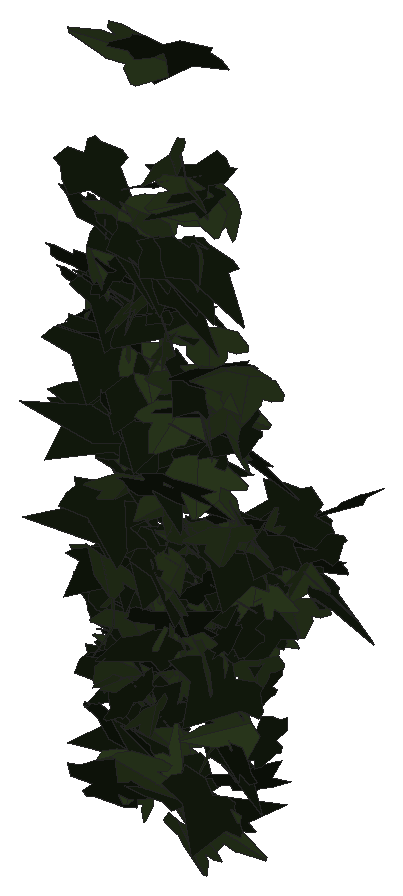
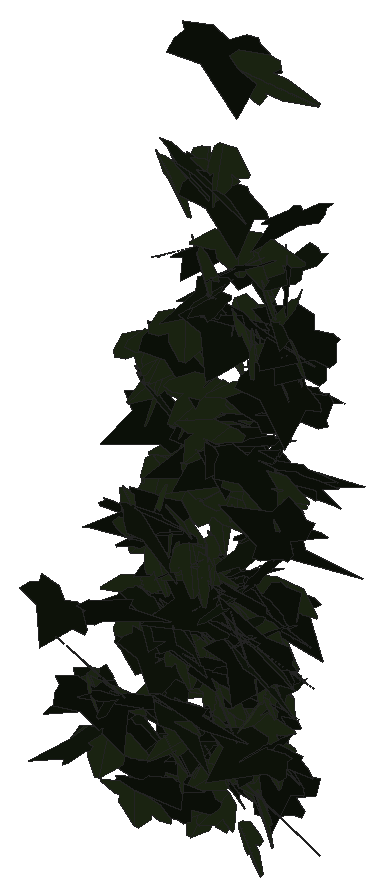
# SketchUp Ruby script. Lengths in millimetres.
U = 1.mm
M = Sketchup.active_model
def pt(a) = Geom::Point3d.new(a.map { |v| v * U })
def face(e, loops, mat)
  f = e.add_face(loops[0].map { |a| pt(a) })
  loops[1..].each { |l| e.add_face(l.map { |a| pt(a) }).erase! }
  f.material = f.back_material = mat if mat
  f
end
# faces: each face lists its corners as indices into pts; further lists are holes
def faces(e, pts, list, mat = nil) = list.each { |f| face(e, (f[0].is_a?(Array) ? f : [f]).map { |l| l.map { |i| pts[i] } }, mat) }
# xy, xz, yz: faces in a plane at the given z, y or x. An outline is a flat list of corners, or four numbers for a rectangle; further outlines are holes
def ring(l) = l.size == 4 ? [[l[0], l[1]], [l[2], l[1]], [l[2], l[3]], [l[0], l[3]]] : l.each_slice(2).to_a
def flat(e, list, mat, &to3) = list.each { |f| face(e, (f[0].is_a?(Array) ? f : [f]).map { |l| ring(l).map { |u, v| to3.(u, v) } }, mat) }
def xy(e, z, list, mat = nil) = flat(e, list, mat) { |x, y| [x, y, z] }
def xz(e, y, list, mat = nil) = flat(e, list, mat) { |x, z| [x, y, z] }
def yz(e, x, list, mat = nil) = flat(e, list, mat) { |y, z| [x, y, z] }
def lines(e, pts, list) = list.each { |a, b| e.add_line(pt(pts[a]), pt(pts[b])) }
# prism: a flat outline (further loops are holes) pulled along v
def prism(e, loops, v, mat = nil)
  f = face(e, loops, mat); d = Geom::Vector3d.new(v.map { |x| x * U })
  f.pushpull(f.normal.samedirection?(d) ? d.length : -d.length)
end
def box(e, o, s, mat = nil) = prism(e, [[o, [o[0] + s[0], o[1], o[2]], [o[0] + s[0], o[1] + s[1], o[2]], [o[0], o[1] + s[1], o[2]]]], [0, 0, s[2]], mat)
def at(x, y, z, deg = 0) = Geom::Transformation.translation(pt([x, y, z])) * Geom::Transformation.rotation(ORIGIN, Z_AXIS, deg.degrees)
def axes(o, x, y, z) = Geom::Transformation.new([*x, 0, *y, 0, *z, 0, *pt(o).to_a, 1])
def part(name) = M.definitions.add(name)
# library, detail: a bought-in or finely detailed component or shape, given as its bounding box
def library(name, o, s) = part(name).tap { |d| box(d.entities, o, s) }
def detail(e, o, s) = box(e.add_group.entities, o, s)
def put(e, d, t, mat = nil) = e.add_instance(d, t).tap { |i| i.material = mat if mat }
def group(e, t, mat = nil) = e.add_group.tap { |g| g.transformation = t; g.material = mat if mat }.entities
root = M.entities
M.materials.add("efeu1").color = [18, 25, 13]
M.materials.add("efeu2").color = [43, 57, 29]
c1 = part("ivyleaf_10")
p = [[0,12.8,-0.8],[-1.5,51.3,-10.9],[-4.9,51,-11.6],[-13.6,26.5,-7.3],[-13.2,15.9,-4.6],[-21.1,19.3,-7.2],
  [-29.5,16.3,-8.3],[-29.2,8.3,-6.2],[-19.7,-9.8,0.5],[-7.6,-13,4],[1,-12.2,5.8],[-0.4,51.1,-11.1],
  [-1.5,51.1,-10.9],[1,-12.4,5.9],[16.9,-12.4,3.5],[35.1,9.1,-5.1],[35,12.9,-6.1],[20.5,16.4,-4.9],
  [15.8,15,-3.8],[15.3,27.6,-7.1],[12.8,31.3,-7.8]]
faces(c1.entities,p,[[0,1,2,3,4,5,6,7,8,9,10],[11,12,0,13,14,15,16,17,18,19,20]],"efeu2")
c2 = part("ivyleaf_9")
p = [[39.1,54.8,31.7],[34.5,51.8,30.2],[-5.3,25.2,17.3],[-17.9,28.3,20.9],[-21.6,21.7,17],[-20.2,4.3,5.3],
  [-22.9,-0.3,2.5],[-17.1,-4,-0.6],[-2,-2.1,-1.2],[-0.7,-15.4,-10.1],[16.6,-22.3,-16.7],[21.1,-15.1,-12.5],
  [32.7,-10.7,-11],[46.1,-1.8,-6.6],[30.8,11.2,3.8]]
faces(c2.entities,p,[[0,1,2,3,4,5,6,7,8,9,10,11,12,13,14]],"efeu1")
put(root,c1,axes([3466.4,1094.4,1814.6],[0.66107,-0.27488,0.78256],[-1.07318,0.54392,0.44135],[-1.15765,-0.6612,0.03773]))
put(root,c1,axes([3457.1,940.4,1772.6],[-0.12385,-0.86588,-0.03723],[-0.00775,0.03764,-0.8683],[1.64945,-0.06484,-0.00688]))
put(root,c1,axes([3457.4,953.5,1707.4],[0.6326,-0.73908,-0.31298],[-0.1515,0.30673,-0.80886],[1.52,0.33816,0.04964]))
put(root,c1,axes([3455.3,951.2,1865.6],[0.03371,-0.87373,0.07357],[0.08152,-0.07263,-0.87294],[1.66678,0.02123,0.04121]))
put(root,c1,axes([3458.5,971.3,1821.6],[-0.31671,0.98973,0.28837],[0.01159,-0.29115,1.0028],[1.96195,0.16149,0.04063]))
put(root,c2,axes([3438.4,973.8,1791.8],[1.58658,0.21997,0.0242],[-0.07633,0.24291,-0.82662],[-0.4142,0.79783,0.245]))
put(root,c2,axes([3440.1,960.9,1790.2],[0.42613,-0.71473,-0.43281],[-0.22247,0.41688,-0.7489],[1.57461,0.25232,0.01132]))
put(root,c2,axes([3461.6,912.7,2227.3],[0.50914,0.91147,-0.06237],[-0.04838,-0.05754,-0.94988],[-1.73809,0.2686,0.00817]))
put(root,c2,axes([3435.4,935.3,2045.1],[0.09466,-0.1674,1.02834],[1.60341,0.61216,0.0589],[-1.16661,0.82778,0.16439]))
put(root,c2,axes([3481,935.6,1705.2],[-1.31145,0.58055,0.11951],[-0.17523,0.07621,-0.90103],[-1.11438,-0.6952,0.00103]))
put(root,c2,axes([3438.7,889.6,2291.9],[1.81947,0.10212,-0.10441],[-0.20003,0.00093,-0.96137],[-0.19302,0.96169,0.01202]))
put(root,c1,axes([3458.2,895.3,2265.1],[0.79575,-0.87537,-0.0637],[0.11662,0.0995,-0.96514],[1.66634,0.41107,0.09797]))
put(root,c2,axes([3475.2,901,2097.9],[-1.61069,-0.33405,0.13391],[-0.20176,-0.09561,-0.9085],[0.65456,-0.85148,0.04948]))
put(root,c2,axes([3438.9,935.5,1844.6],[0.56183,-0.80922,0.10957],[0.08457,-0.10042,-0.86136],[1.55186,0.29844,0.00727]))
put(root,c2,axes([3484.3,951.5,1887.9],[-0.85841,0.74102,0.15174],[-0.17072,0.12302,-0.8674],[-1.42941,-0.4597,0.01247]))
put(root,c2,axes([3471.6,911.1,2116.1],[-1.52179,-0.47085,-0.07469],[0.11651,0.04323,-0.92791],[0.8998,-0.80191,-0.00616]))
put(root,c2,axes([3447.9,893,2265.4],[1.7974,0.04045,-0.16656],[-0.32194,0.0696,-0.94224],[-0.05259,0.95645,0.07561]))
put(root,c1,axes([3482.9,943.9,1801.6],[-1.48368,-0.21492,0.37094],[-0.64817,-0.15707,-0.80676],[0.49556,-0.84891,0.05536]))
put(root,c2,axes([3461.5,951.7,1893.9],[1.13755,0.63776,-0.01348],[-0.0143,-0.01144,-0.87406],[-1.21396,0.59775,-0.00234]))
put(root,c2,axes([3474.9,890.6,2331.8],[0.05618,-0.38642,0.96852],[0.32609,0.95754,0.37682],[-1.95761,0.14841,0.09056]))
put(root,c2,axes([3457.4,945.7,1778.8],[-1.11658,-0.31593,-0.59243],[1.00708,0.26668,-0.66623],[0.78651,-0.78997,0.01202]))
put(root,c2,axes([3504.7,900.5,2094.2],[-0.85534,0.0005,0.89544],[-1.70415,0.00788,-0.44941],[-0.01383,-1.00186,-0.00308]))
put(root,c2,axes([3483.9,937.3,1779.2],[-1.34557,0.44443,-0.24847],[0.3563,-0.16849,-0.83407],[-0.90118,-0.73021,0.04123]))
put(root,c2,axes([3486.5,1075.5,1872.7],[-0.51206,0.8534,0.01063],[-0.00739,0.00993,-0.89481],[-1.62431,-0.26908,0.00072]))
put(root,c1,axes([3485.3,927.7,2061.8],[-1.30585,0.51321,0.36316],[-0.82301,0.00496,-0.82403],[-0.86856,-0.7763,0.23482]))
put(root,c2,axes([3499,944.4,1906.5],[-1.33243,0.49631,0.19101],[-0.44604,-0.00448,-0.84735],[-0.90853,-0.72567,0.13587]))
put(root,c2,axes([3494.8,938,1910.1],[-0.69503,0.75552,0.27273],[-0.37155,0.20713,-0.83519],[-1.48289,-0.40601,0.08143]))
put(root,c1,axes([3467.3,935.5,1770.4],[-1.28992,0.5337,-0.11149],[0.1588,-0.07425,-0.86265],[-1.02545,-0.68285,0.00666]))
put(root,c2,axes([3479.9,910.1,1727.2],[1.31256,0.055,-0.739],[-1.40946,0.01515,-0.69],[-0.0503,1.01071,0.05055]))
put(root,c2,axes([3501.9,1078.5,1871],[-1.49103,-0.0887,0.43046],[-0.82128,-0.01164,-0.78777],[0.15867,-0.89383,-0.03246]))
put(root,c1,axes([3466.4,1077.7,1845.2],[0.12383,0.40628,0.79383],[0.09893,0.79286,-0.41004],[-1.6943,0.07599,0.03407]))
put(root,c1,axes([3471.2,879.9,2311],[-0.17059,0.96019,0.05758],[-0.08437,0.05364,-0.96357],[-1.82877,-0.09204,0.03908]))
put(root,c2,axes([3492,902.7,1937.9],[0.35176,0.5254,-0.84591],[-0.46686,-0.80982,-0.55658],[-1.83679,0.30645,-0.02053]))
put(root,c2,axes([3459.2,948.5,1894.7],[-0.77804,0.31836,0.72354],[0.99578,-0.50162,0.51634],[1.12773,0.66258,0.04325]))
put(root,c1,axes([3482.8,882.6,1939],[-1.69522,0.24427,0.11586],[-0.20959,0.0365,-0.92359],[-0.46991,-0.89748,-0.00603]))
put(root,c2,axes([3510.5,881.1,1992.5],[-1.40708,0.08568,0.56516],[-1.08066,-0.00366,-0.74224],[-0.1253,-0.93058,0.05495]))
put(root,c2,axes([3486,928.2,1809.2],[0.66578,0.70164,-0.38547],[-0.3964,-0.32641,-0.78316],[-1.47114,0.40548,0.03657]))
put(root,c1,axes([3481.1,923,2099.1],[-1.56203,-0.4387,-0.06342],[0.10327,0.03301,-0.93062],[0.83726,-0.82252,-0.00353]))
put(root,c2,axes([3462.9,875.8,2429.3],[0.33278,-0.71635,-0.68512],[-0.21791,0.67644,-0.7365],[1.8739,0.20588,0.03602]))
put(root,c2,axes([3468,944.6,1913.4],[-0.24833,-0.88076,0.08198],[-0.01661,-0.08158,-0.89037],[1.68344,-0.13073,0.00331]))
put(root,c2,axes([3478,889.5,2203.8],[-1.25693,-0.65762,-0.18862],[0.28098,0.11899,-0.9318],[1.27137,-0.67645,0.01946]))
put(root,c2,axes([3489.4,946.6,1831.1],[-1.60642,-0.19522,-0.12449],[0.2579,-0.03492,-0.86399],[0.35732,-0.85248,0.0639]))
put(root,c2,axes([3466.6,945.9,1872.4],[-0.50895,-0.68197,-0.50877],[0.33179,0.47808,-0.73246],[1.58497,-0.31907,-0.01004]))
put(root,c2,axes([3454.5,899.9,2181.5],[1.96184,0.17194,0.04386],[-0.08435,-0.00091,1.04503],[0.32701,-1.03174,0.00639]))
put(root,c2,axes([3463.8,930,2051.4],[0.27496,-0.90416,0.10259],[0.0317,-0.10123,-0.91563],[1.73155,0.14543,0.00047]))
put(root,c1,axes([3476.1,920.4,2082.4],[1.53615,0.45763,-0.05627],[-0.09344,-0.0275,-0.92785],[-0.87254,0.80863,0.00029]))
put(root,c2,axes([3454.6,889.3,2363.5],[0.68678,-0.89036,0.19543],[0.39221,-0.12506,-0.95029],[1.68996,0.39086,0.14113]))
put(root,c2,axes([3490.9,928.1,1968.9],[-0.42196,-0.14264,0.88694],[-0.85321,-0.77409,-0.23656],[1.4816,-0.4864,0.11637]))
put(root,c1,axes([3489.8,939.1,1770.9],[-0.84583,-0.77722,-0.01084],[0.00326,0.01151,-0.8953],[1.47934,-0.44441,-0.00422]))
put(root,c1,axes([3496.9,931.1,1645],[0.60382,-0.39757,-0.70294],[-0.54341,0.65124,-0.4972],[1.43772,0.41312,0.1073]))
put(root,c2,axes([3498.9,874.7,2293.7],[0.00966,0.63079,0.83793],[0.02259,0.83785,-0.6308],[-1.99598,0.01254,-0.00308]))
put(root,c1,axes([3493,876.8,1869.5],[0.13635,-0.73017,-0.69798],[-0.14289,0.69395,-0.73366],[1.91713,0.10365,-0.00504]))
put(root,c1,axes([3478.9,902.2,1812.7],[-0.47946,-0.54666,-0.73995],[0.66967,0.65161,-0.60119],[1.61778,-0.43174,0.02956]))
put(root,c2,axes([3465,956.5,1752.4],[1.08917,-0.37026,-0.54546],[0.90555,-0.26799,0.68112],[-0.86847,-0.74378,0.02612]))
put(root,c2,axes([3499.5,924.8,2122.5],[0.07204,0.86944,-0.33901],[-0.01192,-0.33905,-0.87023],[-1.77603,0.03754,-0.00791]))
put(root,c2,axes([3478.9,903.5,2249],[-0.47652,-0.80938,0.46528],[0.01651,-0.48372,-0.83679],[1.77672,-0.21258,0.13256]))
put(root,c2,axes([3474.1,903.6,2130.1],[0.6463,-0.73444,-0.50214],[0.97081,-0.27964,0.75397],[-1.38732,-0.53784,0.29368]))
put(root,c2,axes([3518.4,933.3,1944.3],[-1.51851,0.2624,0.30518],[-0.54749,0.10211,-0.83989],[-0.53573,-0.84812,-0.0067]))
put(root,c2,axes([3507.5,896.3,1772.7],[-0.28638,0.76761,0.52063],[-0.17061,0.51293,-0.78217],[-1.75698,-0.17493,-0.00891]))
put(root,c2,axes([3489.8,928.5,1799.4],[0.91461,0.72319,-0.05557],[-0.06659,-0.04346,-0.86828],[-1.37882,0.48181,0.00507]))
put(root,c1,axes([3490.9,898.9,2221.3],[1.13867,-0.73894,-0.21917],[-0.00204,0.27665,-0.93568],[1.46691,0.57398,0.16883]))
put(root,c1,axes([3488.5,957.1,1766.2],[-0.88204,-0.73351,-0.0827],[0.43473,-0.04965,-0.83966],[1.33591,-0.46815,0.21863]))
put(root,c1,axes([3500.9,895.4,2038.5],[-0.59498,-0.83811,0.26236],[-0.17645,-0.24543,-0.89451],[1.66207,-0.32608,-0.00105]))
put(root,c1,axes([3496,910.7,2247.1],[0.00083,-0.93504,-0.1991],[0.08532,0.1989,-0.93401],[1.81747,-0.00891,0.04394]))
put(root,c2,axes([3522,950.5,1907.3],[-1.584,0.17303,0.21694],[-0.42658,-0.01484,-0.84808],[-0.31134,-0.85996,0.05829]))
put(root,c2,axes([3487.8,888.7,2016.2],[-0.69692,-0.84517,-0.20789],[0.15481,0.19133,-0.92108],[1.64922,-0.37511,-0.00139]))
put(root,c1,axes([3498.2,892.9,2321],[0.6508,-0.90255,-0.20089],[-0.00172,0.21386,-0.96236],[1.75976,0.33399,0.07335]))
put(root,c2,axes([3487.2,915.2,1945.2],[-1.06426,0.00614,-0.72735],[1.36407,-0.1518,-0.55231],[-0.23607,-0.90482,0.08772]))
put(root,c1,axes([3500.1,943.8,1919.6],[0.46499,-0.858,-0.093],[-0.00562,0.09583,-0.89181],[1.64251,0.24323,0.02328]))
put(root,c2,axes([3503.6,1103.9,1786],[-1.31859,-0.56153,-0.02279],[0.01993,0.02326,-0.89174],[1.0694,-0.69281,-0.01148]))
put(root,c1,axes([3488.6,925.8,1919.8],[-1.55964,0.13079,-0.38359],[0.58579,-0.36207,-0.781],[-0.50177,-0.82921,0.28052]))
put(root,c1,axes([3503.7,963.8,1823.8],[0.51665,-0.82407,-0.00815],[-0.00893,0.00704,-0.86763],[1.56841,0.2715,-0.00226]))
put(root,c2,axes([3517.8,947.9,1719.5],[0.10858,0.27212,0.82938],[-0.30903,0.81995,-0.25785],[-1.63227,-0.13714,0.10399]))
put(root,c1,axes([3519.6,888.9,2368.5],[-1.66021,-0.29938,0.29897],[-0.53069,-0.10846,-0.9222],[0.60562,-0.91574,0.01148]))
put(root,c2,axes([3503.7,908.4,2167.4],[-1.1127,-0.7611,-0.0035],[0.1745,-0.06604,-0.95306],[1.43799,-0.58092,0.11294]))
put(root,c2,axes([3486.7,925.9,2012.6],[1.18296,-0.55565,-0.384],[-0.31384,0.38122,-0.81855],[1.24658,0.62327,0.15832]))
put(root,c1,axes([3542.9,873.5,2581.4],[0.33263,-0.02371,-1.04456],[-1.92406,0.26363,-0.17513],[0.5022,1.02575,0.02087]))
put(root,c2,axes([3484.5,942.2,1915.7],[0.79957,-0.78906,0.09861],[0.10497,-0.08234,-0.89388],[1.50978,0.42361,0.00993]))
put(root,c1,axes([3502.2,895.2,1698.8],[1.25553,0.57269,-0.04042],[-0.05812,-0.02648,-0.8736],[-1.09112,0.6604,0.00002]))
put(root,c1,axes([3508.2,899,1871.2],[-1.57248,-0.33268,-0.21949],[0.37467,0.09862,-0.89052],[0.65955,-0.84918,-0.01743]))
put(root,c2,axes([3549.3,893.9,2274.4],[-1.03988,0.47653,0.63127],[-1.00388,0.35218,-0.7224],[-1.12169,-0.75697,0.0613]))
put(root,c1,axes([3514.5,895.1,2260],[0.46297,-0.88016,-0.33975],[0.1027,0.36327,-0.90244],[1.79264,0.2065,0.13944]))
put(root,c2,axes([3477.9,943.9,1841.6],[0.84895,-0.24546,0.70342],[1.31545,-0.16966,-0.4975],[0.52922,0.81547,0.10823]))
put(root,c2,axes([3479.5,872.4,1673.9],[0.66541,0.01544,0.92468],[1.75756,0.04718,-0.34996],[-0.09438,0.98744,0.00227]))
put(root,c1,axes([3505.2,1116.3,1769.8],[1.64105,-0.13101,0.18554],[0.34997,-0.0249,-0.87215],[0.25373,0.88164,0.00294]))
put(root,c1,axes([3521.7,871.1,2271.3],[0.07225,-0.90385,-0.38317],[0.03306,0.38401,-0.90412],[1.86811,0.02816,0.03082]))
put(root,c2,axes([3520.8,908.6,2127.1],[-0.79224,-0.8496,0.05665],[-0.02772,-0.05594,-0.94602],[1.62031,-0.41636,0.01152]))
put(root,c1,axes([3522.1,953.8,1788.4],[1.25258,-0.58268,0.02379],[0.15652,0.05722,-0.87361],[1.09878,0.65608,0.09733]))
put(root,c1,axes([3529.8,904.1,1768.3],[-0.19956,-0.88455,-0.2076],[0.08031,0.20401,-0.89057],[1.72735,-0.11168,0.01742]))
put(root,c2,axes([3514.5,890.6,2347.9],[-0.37382,-0.93581,-0.22969],[0.12451,0.22092,-0.95603],[1.82967,-0.20623,0.01813]))
put(root,c2,axes([3549.5,899.2,1865.5],[-1.61723,0.41026,-0.04875],[0.0827,-0.02213,-0.94359],[-0.78193,-0.85085,0.00103]))
put(root,c1,axes([3520.9,900.6,2196.1],[0.78011,0.86251,-0.02569],[-0.02298,-0.02271,-0.95495],[-1.64209,0.41007,0.00116]))
put(root,c1,axes([3519.3,952.1,1827.5],[1.50543,-0.38237,0.07111],[0.33703,0.2106,-0.8374],[0.65902,0.76576,0.26581]))
put(root,c2,axes([3517.6,931.5,1759.9],[0.35138,0.11111,-0.87116],[-0.2708,0.88223,0.08236],[1.64934,0.12118,0.19912]))
put(root,c1,axes([3535.8,891,2284.4],[0.10788,-0.97046,-0.11411],[-0.04078,0.11304,-0.972],[1.85926,0.05879,-0.0147]))
put(root,c2,axes([3527.6,916.3,1957.5],[-0.68784,-0.85485,0.15106],[-0.06743,-0.14896,-0.92778],[1.65079,-0.36228,0.02504]))
put(root,c1,axes([3523.8,927.2,1722.1],[-1.3529,-0.23411,-0.49745],[0.89365,0.16444,-0.74837],[0.54428,-0.8519,-0.00776]))
put(root,c1,axes([3534.8,901.8,2381.1],[1.28932,0.69462,-0.04585],[-0.25258,0.06607,-0.95997],[-1.30057,0.67578,0.14099]))
put(root,c2,axes([3554.7,901.3,2268.9],[-1.53744,-0.49938,0.1584],[-0.20802,-0.12406,-0.94853],[0.97514,-0.8138,0.0474]))
put(root,c2,axes([3537.5,893.5,2134],[1.00478,0.75081,0.22186],[0.1802,0.20439,-0.91702],[-1.47909,0.53494,0.03899]))
put(root,c2,axes([3520.3,942,1935.3],[0.92397,-0.72651,-0.21607],[0.01167,0.26034,-0.86161],[1.4425,0.46325,0.14537]))
put(root,c1,axes([3519.5,872.3,1711.8],[-1.09455,-0.04177,-0.72546],[1.3691,0.09804,-0.57593],[0.19548,-0.92056,-0.02842]))
put(root,c2,axes([3539.8,1108,1883.1],[-0.98194,-0.673,-0.22751],[0.27633,0.17535,-0.84798],[1.32353,-0.53592,0.00825]))
put(root,c2,axes([3526.3,909.2,2077.4],[0.17009,-1.07301,0.08296],[0.02119,-0.08232,-1.07672],[2.04815,0.08996,0.00425]))
put(root,c2,axes([3527.2,913.5,2109],[1.76037,0.13837,-0.00241],[-0.03188,0.09577,-0.93018],[-0.26144,0.91998,0.0972]))
put(root,c2,axes([3575.8,902.7,1692.1],[-1.60471,-0.36222,-0.24054],[-0.38881,-0.13328,0.91678],[-0.73051,0.86662,0.04045]))
put(root,c2,axes([3552.6,906.1,2128.6],[0.75669,0.83244,-0.21397],[-0.22977,-0.17933,-0.922],[-1.61958,0.41437,0.03083]))
put(root,c1,axes([3555.8,923.7,1985.2],[0.44518,-0.34468,-0.80439],[-0.30641,0.80146,-0.39024],[1.63711,0.24373,0.1457]))
put(root,c2,axes([3535,891.7,2340.8],[-0.20827,-0.97813,0.07502],[-0.00071,-0.07545,-0.9842],[1.86704,-0.10914,0.008]))
put(root,c2,axes([3545.6,891.8,2260.1],[0.92668,0.817,0.23185],[0.14536,0.22405,-0.94989],[-1.60976,0.49055,0.04769]))
put(root,c1,axes([3545.2,921,1918.5],[1.64832,-0.24935,-0.03911],[-0.06902,0.0154,-0.90125],[0.47539,0.86682,0.00476]))
put(root,c2,axes([3561.9,888.3,2427.9],[0.45116,0.94658,0.0071],[-0.29776,0.0464,-0.96209],[-1.77679,0.23257,0.16303]))
put(root,c1,axes([3543.4,920.5,1668.9],[-1.32058,0.55552,-0.2453],[0.33594,-0.17188,-0.88856],[-1.10586,-0.7156,0.023]))
put(root,c1,axes([3569.3,909,2042.9],[-0.8531,-0.6664,0.65634],[-0.6422,-0.56359,-0.80268],[1.66026,-0.56041,0.02677]))
put(root,c2,axes([3548.8,958.1,1862],[-1.19762,-0.54802,-0.2724],[0.49335,0.11524,-0.83067],[1.05507,-0.67594,0.07922]))
put(root,c2,axes([3531.2,943.9,1924.1],[1.33516,0.27035,0.45747],[0.66417,0.33696,-0.73429],[-0.76266,0.76673,0.1614]))
put(root,c2,axes([3543.5,917.4,1943.5],[-0.25927,-0.89265,0.25627],[0.04945,-0.26258,-0.9008],[1.76683,-0.12364,0.06282]))
put(root,c1,axes([3550.6,923.8,1900.5],[0.29463,-0.78586,0.41306],[0.43913,-0.36928,-0.78902],[1.6316,0.24129,0.13777]))
put(root,c2,axes([3566.1,946.1,1774.2],[0.62675,0.80594,0.12343],[-0.35786,0.2046,-0.83427],[-1.50992,0.28605,0.24896]))
put(root,c1,axes([3560.1,1100.9,1819.7],[-1.36199,-0.52511,-0.14065],[0.23056,0.07263,-0.88753],[1.00861,-0.7257,0.01295]))
put(root,c1,axes([3551,916.2,1862.9],[-0.09025,-0.87433,0.09197],[0.60638,-0.10293,-0.81428],[1.55946,-0.01058,0.32195]))
put(root,c1,axes([3562.4,905.2,2136.3],[1.24198,0.57554,-0.37706],[-0.56097,-0.23575,-0.86996],[-1.18328,0.71586,0.01666]))
put(root,c1,axes([3577.1,885.1,2017.5],[-1.23217,0.41756,0.57915],[-0.89568,0.33834,-0.77004],[-1.02187,-0.80005,-0.02339]))
put(root,c2,axes([3543.3,948.4,1931.4],[0.34069,-0.86299,-0.10728],[-0.01489,0.10792,-0.88124],[1.65501,0.17862,0.01415]))
put(root,c1,axes([3546,917,2135.3],[0.8895,0.61433,0.53449],[0.36912,0.51455,-0.76101],[-1.50517,0.48923,0.12923]))
put(root,c1,axes([3563.3,910.8,1701.3],[0.19651,0.88613,-0.27267],[0.06383,0.27061,0.89213],[1.76337,-0.10855,-0.00191]))
put(root,c1,axes([3563.6,935.7,1972.3],[1.19654,-0.54632,-0.36655],[-0.12454,0.45257,-0.78676],[1.24589,0.56992,0.27339]))
put(root,c2,axes([3575.6,1103.8,1877.5],[0.51464,0.71689,-0.42514],[-0.56351,-0.33517,-0.75352],[-1.48279,0.37619,0.13881]))
put(root,c1,axes([3567.3,941.8,1981.9],[-0.62656,-0.82957,-0.13957],[0.08803,0.1318,-0.89249],[1.5986,-0.3324,-0.00556]))
put(root,c1,axes([3566.1,883.5,2239.3],[0.4688,-0.93465,0.15357],[0.02795,-0.15489,-0.96624],[1.80246,0.2455,-0.02496]))
put(root,c2,axes([3570.7,950.4,1885],[0.32092,0.24229,0.83571],[0.05712,0.84913,-0.25223],[-1.65504,0.07629,0.15334]))
put(root,c1,axes([3594.7,938.6,1968.1],[0.34497,-0.00387,-0.88794],[-1.65245,0.18906,-0.17806],[0.354,0.88631,0.03411]))
put(root,c1,axes([3559.5,932,1959.2],[0.96271,0.7239,-0.12618],[-0.11186,-0.11283,-0.88298],[-1.39403,0.50898,-0.01628]))
put(root,c2,axes([3572.4,869,2604.5],[1.12801,0.74385,-0.47283],[-0.54019,-0.37837,-0.95103],[-1.58815,0.65703,-0.01236]))
put(root,c2,axes([3540.1,899.4,1877.1],[1.61971,0.44597,-0.04084],[0.04214,0.0457,0.96034],[0.85129,-0.8508,0.03017]))
put(root,c1,axes([3560.2,888.1,1932.2],[-0.98501,0.7016,-0.18904],[0.24227,-0.14095,-0.87165],[-1.36152,-0.53267,-0.01834]))
put(root,c1,axes([3572.5,948.6,1865.5],[-0.55997,-0.83577,-0.04837],[0.02997,0.04574,-0.88605],[1.59303,-0.29465,-0.00033]))
put(root,c1,axes([3570.4,879.9,2463.1],[-0.21051,-0.90914,-0.53316],[0.22707,0.52184,-0.91459],[1.99297,-0.15549,0.04789]))
put(root,c2,axes([3577.6,918.2,2113.3],[-1.68507,-0.12323,-0.29911],[0.56315,0.04381,-0.89392],[0.24886,-0.93352,-0.00246]))
put(root,c1,axes([3565.5,1091.6,1874.1],[1.6731,-0.05705,0.01339],[0.04198,0.13566,-0.87026],[0.10333,0.86867,0.13679]))
put(root,c2,axes([3537.5,921.5,1944.7],[1.15445,-0.54381,0.3875],[0.8341,-0.07075,-0.78533],[0.95882,0.71631,0.21662]))
put(root,c1,axes([3571.5,870.7,2252.9],[0.60075,-0.74545,-0.55087],[0.21319,0.60835,-0.75905],[1.75115,0.18167,0.28139]))
put(root,c1,axes([3572.7,888.2,1963.7],[1.08049,-0.73605,0.04453],[0.04579,-0.03767,-0.92955],[1.40267,0.56822,-0.00395]))
put(root,c1,axes([3562.4,909.7,2180.8],[-1.42486,-0.53494,-0.57908],[0.93357,0.30908,-0.9197],[1.17457,-0.8946,0.02852]))
put(root,c1,axes([3579.7,935.7,1978.4],[-0.24056,-0.90194,-0.0052],[0.00854,0.00462,-0.91075],[1.71658,-0.12642,0.0038]))
put(root,c2,axes([3585.9,961.3,1899.4],[-0.54416,0.66817,-0.49804],[0.39501,-0.45285,-0.72669],[-1.53607,-0.35315,-0.01044]))
put(root,c2,axes([3558.7,902.4,2303.8],[1.38027,-0.56517,-0.29595],[-0.32293,0.26106,-0.91434],[1.17044,0.73851,0.09673]))
put(root,c1,axes([3583.5,1094.6,1877.1],[0.29709,-0.89623,0.09459],[0.01355,-0.09477,-0.90967],[1.71512,0.15599,-0.0092]))
put(root,c2,axes([3558.6,1141.2,1832.1],[1.00603,-0.70482,-0.18242],[-0.03554,0.21223,-0.87411],[1.38516,0.51735,0.11006]))
put(root,c2,axes([3564,953,1872.4],[0.54363,-0.78976,-0.26353],[-0.03002,0.27343,-0.83651],[1.58426,0.27618,0.07458]))
put(root,c2,axes([3572.2,939.2,1965.5],[-0.21818,-0.89674,0.0292],[-0.00045,-0.02941,-0.90403],[1.70758,-0.11459,0.00349]))
put(root,c2,axes([3558.6,863,2071.8],[1.74621,0.30543,0.28421],[0.50738,0.09896,-0.96697],[-0.61079,0.95541,0.0093]))
put(root,c1,axes([3582.5,896.3,1640.7],[-1.52915,0.49539,-0.05629],[0.08902,-0.03139,-0.9439],[-0.9447,-0.80482,0.00217]))
put(root,c2,axes([3606.1,1075,1955.1],[-1.10496,-0.32676,0.61837],[-1.01363,-0.31434,-0.66615],[0.86275,-0.78781,0.00932]))
put(root,c2,axes([3577.5,908.3,2181.9],[-0.24831,-0.58301,0.7306],[-0.27188,-0.71658,-0.59733],[1.75803,-0.19316,0.01081]))
put(root,c2,axes([3564.4,893,2306.6],[0.65763,-0.91916,-0.07585],[-0.02535,0.07602,-0.98186],[1.75512,0.3455,0.01424]))
put(root,c2,axes([3574.6,891.7,2086.8],[0.21761,0.20457,-0.93331],[-0.25287,0.93424,0.18849],[1.80077,0.10647,0.13925]))
put(root,c2,axes([3602.7,1107,1917.1],[-1.5253,0.21462,-0.30086],[0.48081,-0.20621,-0.82008],[-0.51334,-0.83084,0.12582]))
put(root,c2,axes([3566.7,949.7,1815],[0.45133,-0.66891,0.52929],[0.32481,-0.50105,-0.70968],[1.59059,0.29213,-0.00526]))
put(root,c2,axes([3576,886.8,2349.4],[-0.12255,-0.84508,-0.50202],[0.04463,0.50163,-0.84743],[1.8702,-0.06735,-0.01267]))
put(root,c2,axes([3618.7,882.6,2446.5],[-0.64247,0.84818,0.36437],[-0.56778,0.26691,-0.89771],[-1.66264,-0.4189,0.16577]))
put(root,c1,axes([3590.7,896.8,2341.2],[1.06867,-0.7898,-0.14836],[0.02151,0.18873,-0.96195],[1.52929,0.54926,0.1172]))
put(root,c2,axes([3570.4,1094.6,1876.2],[1.46772,-0.40597,-0.12666],[-0.1612,0.11041,-0.86961],[0.79316,0.77368,0.05764]))
put(root,c1,axes([3606,872.2,2446.7],[-1.01239,0.61068,0.57282],[-0.78921,0.39743,-0.80877],[-1.38437,-0.67316,0.04216]))
put(root,c1,axes([3599.7,916.9,1747.2],[0.12281,-0.59585,-0.75032],[-0.01218,0.75173,-0.59753],[1.82347,0.04515,0.04654]))
put(root,c1,axes([3615.1,874.8,2430],[1.3708,-0.18086,-0.65603],[-1.18916,0.2027,-0.74188],[0.51312,0.95293,0.03329]))
put(root,c1,axes([3607.3,905.5,1860.9],[1.19587,-0.57421,-0.46324],[-0.617,0.33168,-0.85089],[1.2613,0.70668,0.02297]))
put(root,c1,axes([3599.4,907.5,2137.3],[-0.57532,0.89132,-0.01357],[-0.20497,-0.05074,-0.93373],[-1.68413,-0.29831,0.11828]))
put(root,c2,axes([3607.6,950.2,1901.7],[0.43978,0.68548,0.5111],[-0.02507,0.53222,-0.70785],[-1.62713,0.17707,0.14905]))
put(root,c1,axes([3572.5,919.2,2062],[1.3699,0.11011,0.65936],[1.1995,0.21122,-0.72329],[-0.42412,0.95301,0.08412]))
put(root,c2,axes([3622,888.2,2441.2],[-1.47269,0.53138,-0.28784],[0.30041,-0.27369,-0.9296],[-1.11025,-0.77891,0.13027]))
put(root,c2,axes([3610.9,946.9,1845.2],[0.39525,0.79963,0.33369],[-0.01066,0.34437,-0.82175],[-1.64902,0.18944,0.08529]))
put(root,c1,axes([3608.4,902,2249.8],[-1.38405,-0.64057,0.00499],[0.19215,-0.12207,-0.95609],[1.20393,-0.71692,0.15833]))
put(root,c1,axes([3602.2,891.7,2090.2],[1.12103,0.82635,-0.14893],[-0.18513,-0.11354,-1.01471],[-1.58729,0.59686,0.01316]))
put(root,c1,axes([3612.4,944,1969.8],[-0.26794,-0.88216,-0.06887],[0.00503,0.06931,-0.89328],[1.68402,-0.14056,-0.00829]))
put(root,c2,axes([3619.6,891.6,2218],[0.40154,0.90775,-0.17965],[-0.09749,-0.17252,-0.93189],[-1.75844,0.21685,0.01064]))
put(root,c2,axes([3580.4,931.7,1650.1],[-0.02227,-0.16519,0.86926],[1.6454,-0.18713,-0.02392],[0.35836,0.84895,0.16387]))
put(root,c2,axes([3590.4,894,2350.5],[0.27852,-0.94407,-0.24076],[0.32546,0.26457,-0.93349],[1.82546,0.09687,0.20317]))
put(root,c1,axes([3618.1,921.3,2000.8],[-1.73194,0.04005,0.01507],[-0.02856,0.00183,-0.91089],[-0.07627,-0.91014,-0.00117]))
put(root,c2,axes([3608.8,903.2,1689.4],[-0.49894,-0.9,0.43293],[-0.22987,-0.41575,-0.9374],[1.8868,-0.28864,0.00028]))
put(root,c2,axes([3609.7,893.4,1955.9],[-0.20959,0.32552,-0.88746],[-0.42283,0.85953,0.34284],[1.74866,0.24685,-0.02347]))
put(root,c2,axes([3634.9,941.4,2006],[-0.40551,0.87033,-0.00129],[-0.00669,-0.00219,-0.89602],[-1.6564,-0.21306,0.00394]))
put(root,c2,axes([3599.8,940.4,1730.1],[0.39805,-0.85335,0.22357],[0.18074,-0.20665,-0.87761],[1.66914,0.22588,0.04172]))
put(root,c1,axes([3637.8,913.9,1779.5],[0.47067,0.21547,-0.88754],[-1.181,-0.63504,-0.32708],[-1.27543,0.66754,-0.02467]))
put(root,c2,axes([3630.6,913.5,1898.9],[-1.10221,0.47345,-0.48352],[0.72743,-0.29634,-0.74796],[-1.06284,-0.69381,-0.01048]))
put(root,c1,axes([3604.2,898,1857.6],[-0.06744,-0.17673,0.90925],[1.13301,-0.70145,-0.11314],[1.35057,0.57963,0.14032]))
put(root,c2,axes([3641.7,907,1732.8],[0.136,-0.34285,0.88112],[-0.50172,0.84136,0.34876],[-1.72805,-0.27126,-0.03191]))
put(root,c1,axes([3613.8,921.5,2013],[1.22318,-0.56124,0.32236],[0.46187,-0.21217,-0.85325],[1.14193,0.68699,-0.00018]))
put(root,c2,axes([3623.1,942.8,1985.1],[-0.7911,-0.78854,-0.01827],[0.0076,0.01855,-0.89137],[1.50113,-0.41566,-0.00512]))
put(root,c1,axes([3598.4,913.6,1653],[-0.4509,0.06611,-0.90975],[1.51716,-0.44184,-0.23971],[-0.84376,-0.82979,0.05516]))
put(root,c2,axes([3651.7,919.9,1901.5],[-1.30071,0.5681,-0.01902],[0.02793,-0.01209,-0.88872],[-1.08145,-0.68359,-0.00008]))
put(root,c2,axes([3599.9,930.8,2004.1],[1.34678,0.14942,0.5741],[1.03795,0.18778,-0.7211],[-0.44426,0.89168,0.05566]))
put(root,c2,axes([3630.8,1093.6,1967.2],[0.54206,0.7494,0.3799],[0.25637,0.35522,-0.8017],[-1.57838,0.31506,0.00025]))
put(root,c2,axes([3611.5,938.3,1690.7],[1.29879,0.57121,0.1933],[-0.28204,-0.12412,0.88994],[1.1125,-0.69833,-0.00005]))
put(root,c1,axes([3634.3,918.8,2034.3],[-0.98923,0.73445,0.16439],[-0.13452,0.15127,-0.89929],[-1.42606,-0.52374,-0.0292]))
put(root,c1,axes([3633.7,902.9,2212.4],[-1.43946,-0.51273,-0.26013],[0.38856,0.16231,-0.91355],[1.02292,-0.78318,-0.01903]))
put(root,c1,axes([3628.2,931.4,1991.8],[-1.30733,0.54402,-0.25399],[0.39565,-0.14656,-0.87614],[-1.07198,-0.71755,-0.01361]))
put(root,c1,axes([3643.9,887.2,2429],[1.15409,-0.69178,-0.3586],[-0.36488,0.30796,-0.9183],[1.43738,0.63362,0.05481]))
put(root,c2,axes([3645.2,894.2,1848.5],[-1.20918,-0.68062,0.22577],[-0.30755,-0.15798,-0.93102],[1.32965,-0.65549,-0.01003]))
put(root,c1,axes([3635.6,946.8,1927.3],[1.09497,0.6599,-0.15884],[-0.27338,-0.08513,-0.87397],[-1.26253,0.59075,0.05149]))
put(root,c2,axes([3634.2,944.5,1905.7],[-0.80728,-0.75561,-0.222],[0.21656,0.1907,-0.8665],[1.48312,-0.43913,0.00569]))
put(root,c2,axes([3659.5,905.5,2154.6],[-1.40101,0.55613,-0.23962],[0.35481,-0.15073,-0.92256],[-1.09652,-0.75933,0.00763]))
put(root,c2,axes([3635.4,910.4,1988.9],[-0.49719,-0.82563,0.29254],[-0.07363,-0.2941,-0.86458],[1.66543,-0.25948,0.04911]))
put(root,c2,axes([3665.3,939.4,1761.7],[-1.12965,0.66654,-0.05058],[0.0655,-0.03708,-0.89252],[-1.27052,-0.59455,-0.00104]))
put(root,c2,axes([3622.8,913,2124.4],[1.73628,-0.24716,-0.00393],[-0.00721,0.00103,-0.94518],[0.47041,0.9123,0]))
put(root,c1,axes([3642.4,941.9,1993.9],[-0.00394,-0.89541,0.09003],[-0.004,0.09004,0.89541],[-1.71273,0.00185,-0.0023]))
put(root,c1,axes([3654.7,875.5,2038.3],[-0.88008,-0.84291,-0.01694],[-0.00587,0.02101,-0.96134],[1.60454,-0.46226,-0.01281]))
put(root,c1,axes([3638.5,898.2,2172.7],[-0.41036,-0.56493,-0.76325],[0.79313,0.64699,-0.5966],[1.6239,-0.45875,0.09851]))
put(root,c2,axes([3664.9,933.5,1829.5],[-1.02603,0.67101,-0.2361],[0.29365,-0.17888,-0.86071],[-1.32158,-0.5607,-0.00795]))
put(root,c1,axes([3655,886.6,2150.4],[-0.66224,0.69214,0.66915],[-0.5095,0.61389,-0.77419],[-1.75997,-0.43816,-0.02766]))
put(root,c1,axes([3656,905.8,2207.1],[-1.38777,-0.6166,0.08605],[0.03819,-0.15573,-0.94586],[1.18427,-0.71753,0.13134]))
put(root,c2,axes([3655.1,937.3,2006.9],[-1.5062,-0.35926,-0.22467],[0.48029,-0.01727,-0.86133],[0.64782,-0.8225,0.11622]))
put(root,c1,axes([3656.9,922.3,1858.1],[-0.82766,-0.76847,-0.11966],[0.08229,0.113,-0.88281],[1.47789,-0.43666,-0.01786]))
